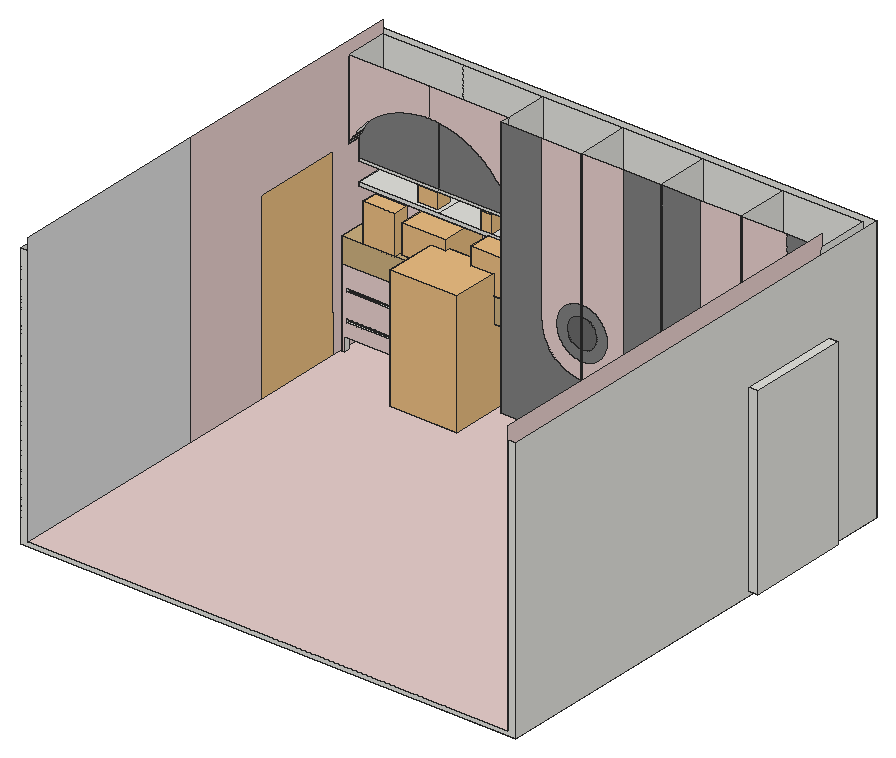
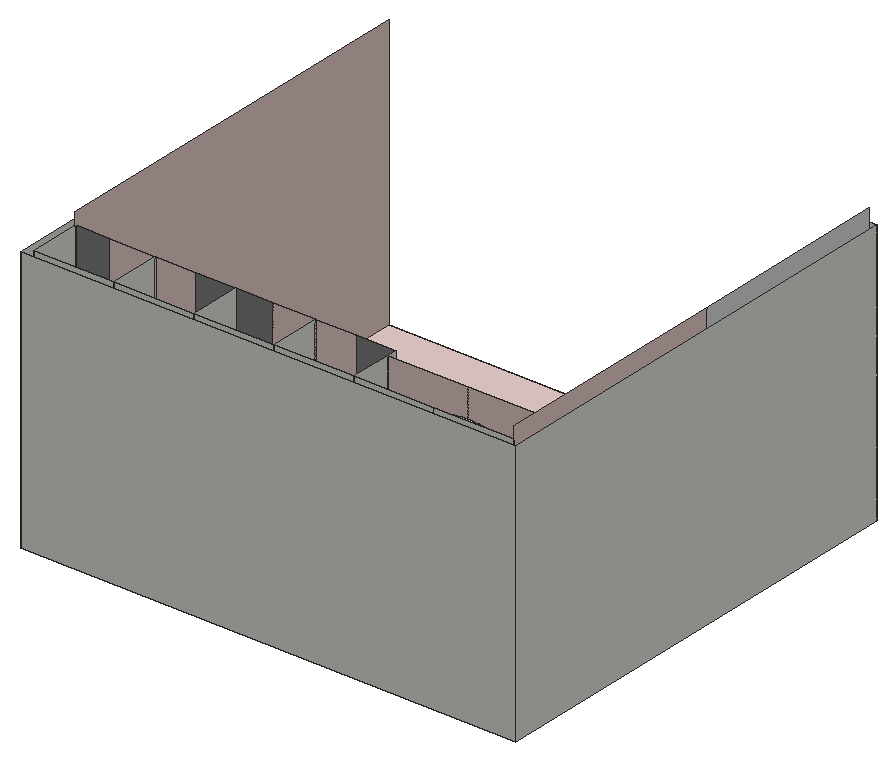
# SketchUp Ruby script. Lengths in inches.
U = 1.inch
M = Sketchup.active_model
def pt(a) = Geom::Point3d.new(a.map { |v| v * U })
def face(e, loops, mat)
  f = e.add_face(loops[0].map { |a| pt(a) })
  loops[1..].each { |l| e.add_face(l.map { |a| pt(a) }).erase! }
  f.material = f.back_material = mat if mat
  f
end
# faces: each face lists its corners as indices into pts; further lists are holes
def faces(e, pts, list, mat = nil) = list.each { |f| face(e, (f[0].is_a?(Array) ? f : [f]).map { |l| l.map { |i| pts[i] } }, mat) }
# xy, xz, yz: faces in a plane at the given z, y or x. An outline is a flat list of corners, or four numbers for a rectangle; further outlines are holes
def ring(l) = l.size == 4 ? [[l[0], l[1]], [l[2], l[1]], [l[2], l[3]], [l[0], l[3]]] : l.each_slice(2).to_a
def flat(e, list, mat, &to3) = list.each { |f| face(e, (f[0].is_a?(Array) ? f : [f]).map { |l| ring(l).map { |u, v| to3.(u, v) } }, mat) }
def xy(e, z, list, mat = nil) = flat(e, list, mat) { |x, y| [x, y, z] }
def xz(e, y, list, mat = nil) = flat(e, list, mat) { |x, z| [x, y, z] }
def yz(e, x, list, mat = nil) = flat(e, list, mat) { |y, z| [x, y, z] }
def lines(e, pts, list) = list.each { |a, b| e.add_line(pt(pts[a]), pt(pts[b])) }
# prism: a flat outline (further loops are holes) pulled along v
def prism(e, loops, v, mat = nil)
  f = face(e, loops, mat); d = Geom::Vector3d.new(v.map { |x| x * U })
  f.pushpull(f.normal.samedirection?(d) ? d.length : -d.length)
end
def box(e, o, s, mat = nil) = prism(e, [[o, [o[0] + s[0], o[1], o[2]], [o[0] + s[0], o[1] + s[1], o[2]], [o[0], o[1] + s[1], o[2]]]], [0, 0, s[2]], mat)
def at(x, y, z, deg = 0) = Geom::Transformation.translation(pt([x, y, z])) * Geom::Transformation.rotation(ORIGIN, Z_AXIS, deg.degrees)
def axes(o, x, y, z) = Geom::Transformation.new([*x, 0, *y, 0, *z, 0, *pt(o).to_a, 1])
def part(name) = M.definitions.add(name)
# library, detail: a bought-in or finely detailed component or shape, given as its bounding box
def library(name, o, s) = part(name).tap { |d| box(d.entities, o, s) }
def detail(e, o, s) = box(e.add_group.entities, o, s)
def put(e, d, t, mat = nil) = e.add_instance(d, t).tap { |i| i.material = mat if mat }
def group(e, t, mat = nil) = e.add_group.tap { |g| g.transformation = t; g.material = mat if mat }.entities
root = M.entities
M.materials.add("[0007_MistyRose]").color = [232, 207, 204]
M.materials.add("[0130_Gainsboro]").color = [220, 220, 220]
M.materials.add("[0133_Gray]").color = [128, 128, 128]
M.materials.add("[0134_DimGray]").color = [105, 105, 105]
M.materials.add("[0136_Charcoal]").color = [35, 35, 35]
M.materials.add("[Wood Floor Light]").color = [204, 176, 127]
c1 = library("skp9D",[0,-0.2,0],[0.48,0.4,0.87])
c2 = part("Group\#2")
detail(c2.entities,[0,0,0],[36,3,84])
c3 = library("Flower+Vase+Glass",[1.07,1.25,0],[13.84,13.38,16.78])
c4 = library("LapTop",[-9.12,-3.35,-0.68],[14.19,15.07,9.17])
c5 = library("Lampe Enna desk ASTRO",[0,0,0],[14.67,7.08,17.81])
c6 = library("ADORNOS+LIVROS+PLANTA+CELULAR+ÓCULOS",[6.19,-1.3125,-0.22],[15.35,11.9,12.07])
c7 = library("Group\#6",[0,0,0],[2.77,2.73,4.26])
xy(root,0,[[0,0,228,207.6875]])
xy(root,2.125,[[3.62,180.25,5.05,183.03],[38.11,180.25,40.45,183.62],[77.27,180.25,114.09,204.25],[114.39,180.25,150.92,180.25,150.92,204.25,114.09,204.25,114.09,180.38,114.39,180.38],[150.92,180.25,187.74,204.25],
  [188.04,180.25,224.57,180.25,224.57,204.25,187.74,204.25,187.74,180.38,188.04,180.38],[3.62,196.71,5.05,196.71,5.05,199.93,40.45,199.93,40.45,204.25,3.62,204.25],[40.45,202.25,77.27,204.25]])
xy(root,2.125,[[[3.43,0,224.57,0,224.57,134,232.38,134,232.38,180.25,188.04,180.25,188.04,180.38,187.74,180.38,187.74,180.25,114.39,180.25,114.39,180.38,114.09,180.38,114.09,180.25,77.27,180.25,77.27,202.25,40.45,202.25,40.45,199.93,5.05,199.93,5.05,196.71,3.62,196.71,3.62,204.25,3.57,175.68,0.14,175.69,0.07,134.44,3.5,134.43,3.43,93.375],[38.11,180.25,40.45,183.62],[3.62,180.25,5.05,183.03]]],"[0007_MistyRose]")
xy(root,8.1875,[[5.05,180.25,5.05,183.03,3.62,183.03,3.62,196.71,5.05,196.71,5.05,199.93,30.74,199.93,30.74,183.62,38.11,183.62,38.11,180.25],[30.74,183.62,40.45,199.93]])
xy(root,14.46,[[5.96,180.25,37.02,181.5]])
xy(root,16.15,[[5.96,180.25,37.02,181.5]])
xy(root,26.96,[[5.96,180.25,37.02,181.5]])
xy(root,28.65,[[5.96,180.25,37.02,181.5]])
xy(root,37.85,[[40.45,180.25,77.27,202.25]])
xy(root,49.45,[[3.62,180.25,77.27,203.88]],"[Wood Floor Light]")
xy(root,65.5,[[3.62,190.13,40.45,203.88],[40.45,190.13,77.27,203.88]])
xy(root,67.29,[[3.62,190.13,40.45,203.88],[40.45,190.13,77.27,203.88]])
xy(root,76.04,[[3.62,190.13,77.27,203.88]])
xy(root,86.125,[[224.57,134,232.38,180.25],[3.5,134.43,0.07,134.44,0.14,175.69,3.57,175.68]])
xz(root,0,[[0,0,228,0,228,122.125,224.57,122.125,224.57,2.125,3.43,2.125,3.43,122.125,0,122.125]])
xz(root,134,[[224.57,2.125,232.38,86.125]])
xz(root,180.25,[[150.92,2.125,151.22,122.125],[114.39,36.55,114.39,41.12,114.09,41.16,114.09,36.59],[187.74,36.6,188.04,36.64,188.04,40.48,187.74,40.44],[187.74,40.44,188.04,40.48,188.04,55.625,187.74,55.67],[114.39,41.12,114.39,54.99,114.09,54.95,114.09,41.16],
  [114.09,54.95,114.39,54.99,114.39,59.55,114.09,59.51],[188.04,55.625,188.04,59.46,187.74,59.5,187.74,55.67]])
xz(root,180.25,[[[3.62,2.125,5.05,2.125,5.05,8.1875,38.11,8.1875,38.11,2.125,40.45,2.125,40.45,37.85,3.62,37.85],[5.96,26.96,37.02,28.65],[5.96,14.46,37.02,16.15]],[224.57,2.125,232.38,86.125],[188.57,28.22,189.1,28.22,189.63,28.23,190.16,28.25,190.6875,28.29,191.21,28.35,191.74,28.41,192.26,28.49,192.79,28.59,193.3,28.7,193.82,28.82,194.33,28.96,194.84,29.11,195.35,29.28,195.85,29.45,196.83,29.85,197.3125,30.07,197.79,30.3,198.26,30.54,198.72,30.8,199.18,31.07,199.63,31.35,200.07,31.64,200.51,31.95,201.35,32.59,201.76,32.93,202.16,33.28,202.55,33.64,203.29,34.4,203.65,34.79,204,35.1875,204.34,35.6,204.98,36.44,205.28,36.88,205.57,37.32,205.85,37.77,206.11,38.23,206.37,38.7,206.61,39.17,206.84,39.65,207.05,40.13,207.26,40.625,207.44,41.12,207.62,41.62,207.78,42.125,207.93,42.63,208.07,43.15,208.1875,43.66,208.29,44.18,208.38,44.71,208.46,45.23,208.53,45.76,208.58,46.29,208.61,46.81,208.63,47.34,208.64,47.875,208.64,122.125,188.04,122.125,188.04,59.46,188.63,59.47,189.22,59.41,189.8,59.32,190.375,59.2,190.95,59.05,191.51,58.87,192.06,58.66,192.6,58.42,193.125,58.16,193.64,57.87,194.14,57.55,194.62,57.21,195.08,56.84,195.52,56.45,195.94,56.04,196.34,55.61,196.72,55.16,197.08,54.6875,197.4,54.2,197.71,53.69,197.98,53.17,198.23,52.64,198.46,52.09,198.65,51.53,198.8125,50.97,198.95,50.39,199.06,49.82,199.13,49.23,199.18,48.64,199.19,48.05,199.18,47.46,199.13,46.875,199.06,46.29,198.95,45.71,198.8125,45.14,198.65,44.57,198.46,44.02,198.23,43.47,197.98,42.9375,197.71,42.42,197.4,41.91,197.08,41.42,196.72,40.95,196.34,40.5,195.94,40.0625,195.52,39.65,195.08,39.26,194.62,38.9,194.14,38.56,193.64,38.24,193.125,37.95,192.6,37.68,192.06,37.45,191.51,37.24,190.95,37.0625,190.375,36.91,189.8,36.79,189.22,36.7,188.63,36.64,188.04,36.64,188.04,28.34],[187.24,28.3,187.74,28.38,187.74,36.6,187.14,36.62,186.54,36.67,185.95,36.74,185.36,36.85,184.78,36.99,184.2,37.16,183.64,37.36,183.08,37.59,182.54,37.85,182.02,38.14,181.51,38.45,181.01,38.79,180.54,39.16,180.08,39.54,179.64,39.96,179.23,40.39,178.84,40.85,178.48,41.32,178.14,41.82,177.83,42.33,177.54,42.86,177.28,43.4,177.05,43.95,176.85,44.52,176.68,45.09,176.54,45.67,176.43,46.26,176.35,46.86,176.31,47.45,176.29,48.05,176.31,48.65,176.35,49.25,176.43,49.84,176.54,50.43,176.68,51.02,176.85,51.59,177.05,52.16,177.28,52.71,177.54,53.25,177.83,53.78,178.14,54.29,178.48,54.78,178.84,55.26,179.23,55.72,179.64,56.15,180.08,56.5625,180.54,56.95,181.01,57.32,181.51,57.66,182.02,57.97,182.54,58.26,183.08,58.51,183.64,58.74,184.2,58.94,184.78,59.11,185.36,59.25,185.95,59.36,186.54,59.44,187.14,59.49,187.74,59.5,187.74,122.125,169.33,122.125,169.33,47.875,169.34,47.38,169.35,46.89,169.39,46.4,169.43,45.9,169.48,45.41,169.55,44.92,169.63,44.4375,169.72,43.95,169.83,43.47,170.07,42.51,170.37,41.57,170.53,41.1,170.71,40.64,170.9,40.1875,171.09,39.73,171.3,39.29,171.76,38.41,172,37.98,172.25,37.56,172.52,37.14,172.79,36.73,173.08,36.33,173.375,35.93,173.68,35.54,173.99,35.16,174.32,34.79,174.65,34.43,174.99,34.07,175.34,33.72,175.7,33.38,176.07,33.06,176.45,32.74,176.83,32.43,177.22,32.125,177.625,31.84,178.03,31.56,178.44,31.29,178.86,31.03,179.29,30.78,179.72,30.54,180.16,30.3125,180.6,30.1,181.05,29.89,181.97,29.51,182.43,29.34,183.37,29.04,183.84,28.9,184.32,28.78,184.8,28.67,185.29,28.57,185.77,28.48,186.26,28.41,186.75,28.35],[114.89,28.5,115.89,28.54,116.39,28.58,116.89,28.64,117.38,28.7,117.875,28.78,118.36,28.875,118.85,28.98,119.34,29.1,119.82,29.23,120.3,29.37,120.77,29.53,121.24,29.7,121.71,29.88,122.17,30.07,123.08,30.49,123.52,30.72,123.96,30.96,124.39,31.21,124.8125,31.48,125.23,31.75,125.64,32.04,126.04,32.33,126.4375,32.64,126.82,32.96,127.2,33.28,127.57,33.62,127.93,33.97,128.28,34.32,128.62,34.6875,128.95,35.0625,129.27,35.44,129.59,35.83,129.89,36.23,130.18,36.64,130.46,37.05,130.72,37.48,130.98,37.9,131.23,38.34,131.46,38.78,131.9,39.68,132.28,40.6,132.62,41.54,132.77,42.02,133.03,42.98,133.14,43.47,133.32,44.45,133.39,44.95,133.45,45.44,133.5,45.94,133.53,46.4375,133.55,46.9375,133.56,47.4375,133.56,122.125,114.39,122.125,114.39,59.55,115,59.54,115.6,59.49,116.19,59.41,116.78,59.3,117.37,59.16,117.95,58.99,118.51,58.79,119.07,58.56,119.61,58.3,120.14,58.01,120.66,57.7,121.15,57.36,121.63,56.99,122.09,56.6,122.53,56.19,122.94,55.75,123.33,55.29,123.7,54.8125,124.04,54.32,124.35,53.8,124.64,53.27,124.9,52.73,125.13,52.17,125.33,51.61,125.5,51.03,125.64,50.44,125.75,49.85,125.83,49.26,125.88,48.66,125.89,48.05,125.88,47.45,125.83,46.85,125.75,46.25,125.64,45.66,125.5,45.08,125.33,44.5,125.13,43.93,124.9,43.375,124.64,42.83,124.35,42.3,124.04,41.79,123.7,41.29,123.33,40.82,122.94,40.36,122.53,39.92,122.09,39.51,121.63,39.12,121.15,38.75,120.66,38.41,120.14,38.09,119.61,37.81,119.07,37.55,118.51,37.32,117.95,37.12,117.37,36.95,116.78,36.8,116.19,36.7,115.6,36.62,115,36.57,114.39,36.55,114.39,28.53],
  [113.61,28.53,114.09,28.57,114.09,36.59,113.5,36.59,112.91,36.65,112.33,36.74,111.75,36.86,111.18,37.01,110.61,37.19,110.06,37.4,109.52,37.64,108.99,37.9,108.47,38.2,107.97,38.51,107.49,38.86,107.02,39.22,106.58,39.62,106.16,40.03,105.75,40.46,105.375,40.92,105.02,41.39,104.6875,41.88,104.38,42.39,104.11,42.91,103.86,43.45,103.63,44,103.4375,44.56,103.27,45.125,103.14,45.7,103.03,46.28,102.95,46.87,102.91,47.46,102.89,48.05,102.91,48.65,102.95,49.24,103.03,49.82,103.14,50.41,103.27,50.98,103.4375,51.55,103.63,52.11,103.86,52.66,104.11,53.19,104.38,53.72,104.6875,54.22,105.02,54.72,105.375,55.1875,105.75,55.64,106.16,56.08,106.58,56.49,107.02,56.88,107.49,57.25,107.97,57.59,108.47,57.91,108.99,58.2,109.52,58.47,110.06,58.7,110.61,58.91,111.18,59.09,111.75,59.25,112.33,59.37,112.91,59.46,113.5,59.52,114.09,59.51,114.09,122.125,95.68,122.125,95.68,47.4375,95.6875,46.95,95.71,46.46,95.74,45.98,95.78,45.49,95.84,45.01,95.91,44.53,95.99,44.05,96.08,43.57,96.1875,43.09,96.3,42.62,96.43,42.15,96.58,41.6875,96.73,41.22,96.9,40.77,97.07,40.3125,97.26,39.86,97.46,39.42,97.67,38.98,98.13,38.12,98.375,37.7,98.63,37.29,98.9,36.88,99.46,36.08,99.76,35.7,100.07,35.32,100.38,34.95,101.04,34.23,101.74,33.55,102.1,33.23,102.47,32.91,102.85,32.6,103.23,32.3,103.625,32.02,104.03,31.74,104.43,31.47,105.27,30.97,105.69,30.73,106.13,30.51,106.57,30.3,107.01,30.1,107.46,29.91,107.91,29.73,108.37,29.5625,108.83,29.41,109.29,29.26,109.76,29.13,110.24,29.01,110.71,28.91,111.1875,28.8125,111.67,28.73,112.15,28.66,112.63,28.6,113.12,28.56]],"[0007_MistyRose]")
xz(root,180.25,[[77.27,2.125,114.09,2.125,114.09,28.57,113.61,28.53,113.12,28.56,112.63,28.6,112.15,28.66,111.67,28.73,111.1875,28.8125,110.71,28.91,110.24,29.01,109.76,29.13,109.29,29.26,108.83,29.41,108.37,29.5625,107.91,29.73,107.46,29.91,107.01,30.1,106.57,30.3,106.13,30.51,105.69,30.73,105.27,30.97,104.43,31.47,104.03,31.74,103.625,32.02,103.23,32.3,102.85,32.6,102.47,32.91,102.1,33.23,101.74,33.55,101.04,34.23,100.38,34.95,100.07,35.32,99.76,35.7,99.46,36.08,98.9,36.88,98.63,37.29,98.375,37.7,98.13,38.12,97.67,38.98,97.46,39.42,97.26,39.86,97.07,40.3125,96.9,40.77,96.73,41.22,96.58,41.6875,96.43,42.15,96.3,42.62,96.1875,43.09,96.08,43.57,95.99,44.05,95.91,44.53,95.84,45.01,95.78,45.49,95.74,45.98,95.71,46.46,95.6875,46.95,95.68,47.4375,95.68,122.125,77.27,122.125],[114.39,2.125,150.92,2.125,150.92,122.125,133.56,122.125,133.56,47.4375,133.55,46.9375,133.53,46.4375,133.5,45.94,133.45,45.44,133.39,44.95,133.32,44.45,133.14,43.47,133.03,42.98,132.77,42.02,132.62,41.54,132.28,40.6,131.9,39.68,131.46,38.78,131.23,38.34,130.98,37.9,130.72,37.48,130.46,37.05,130.18,36.64,129.89,36.23,129.59,35.83,129.27,35.44,128.95,35.0625,128.62,34.6875,128.28,34.32,127.93,33.97,127.57,33.62,127.2,33.28,126.82,32.96,126.4375,32.64,126.04,32.33,125.64,32.04,125.23,31.75,124.8125,31.48,124.39,31.21,123.96,30.96,123.52,30.72,123.08,30.49,122.17,30.07,121.71,29.88,121.24,29.7,120.77,29.53,120.3,29.37,119.82,29.23,119.34,29.1,118.85,28.98,118.36,28.875,117.875,28.78,117.38,28.7,116.89,28.64,116.39,28.58,115.89,28.54,114.89,28.5,114.39,28.53],[151.22,2.125,187.74,2.125,187.74,28.38,187.24,28.3,186.75,28.35,186.26,28.41,185.77,28.48,185.29,28.57,184.8,28.67,184.32,28.78,183.84,28.9,183.37,29.04,182.43,29.34,181.97,29.51,181.05,29.89,180.6,30.1,180.16,30.3125,179.72,30.54,179.29,30.78,178.86,31.03,178.44,31.29,178.03,31.56,177.625,31.84,177.22,32.125,176.83,32.43,176.45,32.74,176.07,33.06,175.7,33.38,175.34,33.72,174.99,34.07,174.65,34.43,174.32,34.79,173.99,35.16,173.68,35.54,173.375,35.93,173.08,36.33,172.79,36.73,172.52,37.14,172.25,37.56,172,37.98,171.76,38.41,171.3,39.29,171.09,39.73,170.9,40.1875,170.71,40.64,170.53,41.1,170.37,41.57,170.07,42.51,169.83,43.47,169.72,43.95,169.63,44.4375,169.55,44.92,169.48,45.41,169.43,45.9,169.39,46.4,169.35,46.89,169.34,47.38,169.33,47.875,169.33,122.125,151.22,122.125],[188.04,2.125,224.57,2.125,224.57,122.125,208.64,122.125,208.64,47.875,208.63,47.34,208.61,46.81,208.58,46.29,208.53,45.76,208.46,45.23,208.38,44.71,208.29,44.18,208.1875,43.66,208.07,43.15,207.93,42.63,207.78,42.125,207.62,41.62,207.44,41.12,207.26,40.625,207.05,40.13,206.84,39.65,206.61,39.17,206.37,38.7,206.11,38.23,205.85,37.77,205.57,37.32,205.28,36.88,204.98,36.44,204.34,35.6,204,35.1875,203.65,34.79,203.29,34.4,202.55,33.64,202.16,33.28,201.76,32.93,201.35,32.59,200.51,31.95,200.07,31.64,199.63,31.35,199.18,31.07,198.72,30.8,198.26,30.54,197.79,30.3,197.3125,30.07,196.83,29.85,195.85,29.45,195.35,29.28,194.84,29.11,194.33,28.96,193.82,28.82,193.3,28.7,192.79,28.59,192.26,28.49,191.74,28.41,191.21,28.35,190.6875,28.29,190.16,28.25,189.63,28.23,189.1,28.22,188.57,28.22,188.04,28.34],[114.39,36.55,115,36.57,115.6,36.62,116.19,36.7,116.78,36.8,117.37,36.95,117.95,37.12,118.51,37.32,119.07,37.55,119.61,37.81,120.14,38.09,120.66,38.41,121.15,38.75,121.63,39.12,122.09,39.51,122.53,39.92,122.94,40.36,123.33,40.82,123.7,41.29,124.04,41.79,124.35,42.3,124.64,42.83,124.9,43.375,125.13,43.93,125.33,44.5,125.5,45.08,125.64,45.66,125.75,46.25,125.83,46.85,125.88,47.45,125.89,48.05,125.88,48.66,125.83,49.26,125.75,49.85,125.64,50.44,125.5,51.03,125.33,51.61,125.13,52.17,124.9,52.73,124.64,53.27,124.35,53.8,124.04,54.32,123.7,54.8125,123.33,55.29,122.94,55.75,122.53,56.19,122.09,56.6,121.63,56.99,121.15,57.36,120.66,57.7,120.14,58.01,119.61,58.3,119.07,58.56,118.51,58.79,117.95,58.99,117.37,59.16,116.78,59.3,116.19,59.41,115.6,59.49,115,59.54,114.39,59.55,114.39,54.99,114.76,54.98,115.12,54.95,115.48,54.91,115.84,54.84,116.1875,54.75,116.54,54.65,116.88,54.53,117.22,54.39,117.54,54.23,117.86,54.0625,118.17,53.87,118.47,53.67,118.76,53.45,119.04,53.21,119.3,52.96,119.55,52.7,119.79,52.42,120.01,52.13,120.21,51.83,120.4,51.52,120.58,51.2,120.73,50.875,120.87,50.54,120.99,50.2,121.09,49.85,121.18,49.5,121.25,49.14,121.29,48.78,121.32,48.42,121.33,48.05,121.32,47.69,121.29,47.33,121.25,46.97,121.18,46.61,121.09,46.26,120.99,45.91,120.87,45.57,120.73,45.23,120.58,44.9,120.4,44.58,120.21,44.28,120.01,43.98,119.79,43.6875,119.55,43.41,119.3,43.15,119.04,42.9,118.76,42.66,118.47,42.44,118.17,42.24,117.86,42.05,117.54,41.87,117.22,41.72,116.88,41.58,116.54,41.46,116.1875,41.35,115.84,41.27,115.48,41.2,115.12,41.15,114.76,41.125,114.39,41.12],
  [113.5,36.59,114.09,36.59,114.09,41.16,113.74,41.15,113.39,41.1875,113.04,41.25,112.7,41.33,112.36,41.42,112.02,41.53,111.69,41.66,111.37,41.81,111.06,41.97,110.75,42.15,110.46,42.34,110.17,42.55,109.9,42.77,109.63,43.01,109.38,43.26,109.15,43.52,108.92,43.79,108.71,44.07,108.52,44.37,108.34,44.67,108.17,44.98,108.02,45.31,107.89,45.63,107.78,45.97,107.68,46.31,107.6,46.65,107.54,47,107.49,47.35,107.47,47.7,107.46,48.05,107.47,48.41,107.49,48.76,107.54,49.11,107.6,49.46,107.68,49.8,107.78,50.14,107.89,50.47,108.02,50.8,108.17,51.12,108.34,51.43,108.52,51.74,108.71,52.03,108.92,52.32,109.15,52.59,109.38,52.85,109.63,53.1,109.9,53.34,110.17,53.56,110.46,53.77,110.75,53.96,111.06,54.14,111.37,54.3,111.69,54.44,112.02,54.57,112.36,54.69,112.7,54.78,113.04,54.86,113.39,54.92,113.74,54.96,114.09,54.95,114.09,59.51,113.5,59.52,112.91,59.46,112.33,59.37,111.75,59.25,111.18,59.09,110.61,58.91,110.06,58.7,109.52,58.47,108.99,58.2,108.47,57.91,107.97,57.59,107.49,57.25,107.02,56.88,106.58,56.49,106.16,56.08,105.75,55.64,105.375,55.1875,105.02,54.72,104.6875,54.22,104.38,53.72,104.11,53.19,103.86,52.66,103.63,52.11,103.4375,51.55,103.27,50.98,103.14,50.41,103.03,49.82,102.95,49.24,102.91,48.65,102.89,48.05,102.91,47.46,102.95,46.87,103.03,46.28,103.14,45.7,103.27,45.125,103.4375,44.56,103.63,44,103.86,43.45,104.11,42.91,104.38,42.39,104.6875,41.88,105.02,41.39,105.375,40.92,105.75,40.46,106.16,40.03,106.58,39.62,107.02,39.22,107.49,38.86,107.97,38.51,108.47,38.2,108.99,37.9,109.52,37.64,110.06,37.4,110.61,37.19,111.18,37.01,111.75,36.86,112.33,36.74,112.91,36.65],[187.74,36.6,187.74,40.44,187.34,40.45,186.95,40.48,186.55,40.54,186.16,40.61,185.77,40.7,185.39,40.81,185.01,40.95,184.65,41.1,184.29,41.27,183.9375,41.46,183.6,41.67,183.27,41.9,182.95,42.14,182.65,42.4,182.36,42.67,182.08,42.96,181.83,43.26,181.58,43.58,181.36,43.91,181.15,44.25,180.96,44.6,180.79,44.96,180.64,45.33,180.5,45.7,180.39,46.08,180.3,46.47,180.22,46.86,180.17,47.26,180.14,47.66,180.13,48.05,180.14,48.45,180.17,48.85,180.22,49.24,180.3,49.64,180.39,50.02,180.5,50.41,180.64,50.78,180.79,51.15,180.96,51.51,181.15,51.86,181.36,52.2,181.58,52.53,182.08,53.15,182.36,53.4375,182.65,53.71,182.95,53.97,183.27,54.21,183.6,54.4375,183.9375,54.65,184.29,54.84,184.65,55.01,185.01,55.16,185.39,55.29,185.77,55.41,186.16,55.5,186.55,55.57,186.95,55.625,187.34,55.65,187.74,55.67,187.74,59.5,187.14,59.49,186.54,59.44,185.95,59.36,185.36,59.25,184.78,59.11,184.2,58.94,183.64,58.74,183.08,58.51,182.54,58.26,182.02,57.97,181.51,57.66,181.01,57.32,180.54,56.95,180.08,56.5625,179.64,56.15,179.23,55.72,178.84,55.26,178.48,54.78,178.14,54.29,177.83,53.78,177.54,53.25,177.28,52.71,177.05,52.16,176.85,51.59,176.68,51.02,176.54,50.43,176.43,49.84,176.35,49.25,176.31,48.65,176.29,48.05,176.31,47.45,176.35,46.86,176.43,46.26,176.54,45.67,176.68,45.09,176.85,44.52,177.05,43.95,177.28,43.4,177.54,42.86,177.83,42.33,178.14,41.82,178.48,41.32,178.84,40.85,179.23,40.39,179.64,39.96,180.08,39.54,180.54,39.16,181.01,38.79,181.51,38.45,182.02,38.14,182.54,37.85,183.08,37.59,183.64,37.36,184.2,37.16,184.78,36.99,185.36,36.85,185.95,36.74,186.54,36.67,187.14,36.62],[188.04,36.64,188.63,36.64,189.22,36.7,189.8,36.79,190.375,36.91,190.95,37.0625,191.51,37.24,192.06,37.45,192.6,37.68,193.125,37.95,193.64,38.24,194.14,38.56,194.62,38.9,195.08,39.26,195.52,39.65,195.94,40.0625,196.34,40.5,196.72,40.95,197.08,41.42,197.4,41.91,197.71,42.42,197.98,42.9375,198.23,43.47,198.46,44.02,198.65,44.57,198.8125,45.14,198.95,45.71,199.06,46.29,199.13,46.875,199.18,47.46,199.19,48.05,199.18,48.64,199.13,49.23,199.06,49.82,198.95,50.39,198.8125,50.97,198.65,51.53,198.46,52.09,198.23,52.64,197.98,53.17,197.71,53.69,197.4,54.2,197.08,54.6875,196.72,55.16,196.34,55.61,195.94,56.04,195.52,56.45,195.08,56.84,194.62,57.21,194.14,57.55,193.64,57.87,193.125,58.16,192.6,58.42,192.06,58.66,191.51,58.87,190.95,59.05,190.375,59.2,189.8,59.32,189.22,59.41,188.63,59.47,188.04,59.46,188.04,55.625,188.43,55.63,188.82,55.59,189.2,55.52,189.58,55.44,189.95,55.34,190.32,55.21,190.68,55.07,191.04,54.91,191.38,54.74,191.72,54.54,192.05,54.33,192.36,54.1,192.66,53.86,192.95,53.6,193.23,53.33,193.49,53.04,193.74,52.74,193.97,52.43,194.18,52.11,194.38,51.77,194.5625,51.43,194.73,51.08,194.87,50.72,195,50.35,195.11,49.98,195.19,49.6,195.26,49.21,195.3125,48.83,195.34,48.44,195.35,48.05,195.34,47.67,195.3125,47.28,195.26,46.89,195.19,46.51,195.11,46.13,195,45.76,194.87,45.39,194.73,45.03,194.5625,44.68,194.38,44.34,194.18,44,193.97,43.68,193.74,43.37,193.49,43.07,193.23,42.78,192.95,42.51,192.66,42.25,192.36,42,192.05,41.78,191.72,41.5625,191.38,41.37,191.04,41.19,190.68,41.03,190.32,40.89,189.95,40.77,189.58,40.67,189.2,40.58,188.82,40.52,188.43,40.47,188.04,40.48]],"[0133_Gray]")
xz(root,180.25,[[187.74,40.44,187.74,55.67,187.34,55.65,186.95,55.625,186.55,55.57,186.16,55.5,185.77,55.41,185.39,55.29,185.01,55.16,184.65,55.01,184.29,54.84,183.9375,54.65,183.6,54.4375,183.27,54.21,182.95,53.97,182.65,53.71,182.36,53.4375,182.08,53.15,181.58,52.53,181.36,52.2,181.15,51.86,180.96,51.51,180.79,51.15,180.64,50.78,180.5,50.41,180.39,50.02,180.3,49.64,180.22,49.24,180.17,48.85,180.14,48.45,180.13,48.05,180.14,47.66,180.17,47.26,180.22,46.86,180.3,46.47,180.39,46.08,180.5,45.7,180.64,45.33,180.79,44.96,180.96,44.6,181.15,44.25,181.36,43.91,181.58,43.58,181.83,43.26,182.08,42.96,182.36,42.67,182.65,42.4,182.95,42.14,183.27,41.9,183.6,41.67,183.9375,41.46,184.29,41.27,184.65,41.1,185.01,40.95,185.39,40.81,185.77,40.7,186.16,40.61,186.55,40.54,186.95,40.48,187.34,40.45],[188.43,40.47,188.82,40.52,189.2,40.58,189.58,40.67,189.95,40.77,190.32,40.89,190.68,41.03,191.04,41.19,191.38,41.37,191.72,41.5625,192.05,41.78,192.36,42,192.66,42.25,192.95,42.51,193.23,42.78,193.49,43.07,193.74,43.37,193.97,43.68,194.18,44,194.38,44.34,194.5625,44.68,194.73,45.03,194.87,45.39,195,45.76,195.11,46.13,195.19,46.51,195.26,46.89,195.3125,47.28,195.34,47.67,195.35,48.05,195.34,48.44,195.3125,48.83,195.26,49.21,195.19,49.6,195.11,49.98,195,50.35,194.87,50.72,194.73,51.08,194.5625,51.43,194.38,51.77,194.18,52.11,193.97,52.43,193.74,52.74,193.49,53.04,193.23,53.33,192.95,53.6,192.66,53.86,192.36,54.1,192.05,54.33,191.72,54.54,191.38,54.74,191.04,54.91,190.68,55.07,190.32,55.21,189.95,55.34,189.58,55.44,189.2,55.52,188.82,55.59,188.43,55.63,188.04,55.625,188.04,40.48],[114.39,41.12,114.76,41.125,115.12,41.15,115.48,41.2,115.84,41.27,116.1875,41.35,116.54,41.46,116.88,41.58,117.22,41.72,117.54,41.87,117.86,42.05,118.17,42.24,118.47,42.44,118.76,42.66,119.04,42.9,119.3,43.15,119.55,43.41,119.79,43.6875,120.01,43.98,120.21,44.28,120.4,44.58,120.58,44.9,120.73,45.23,120.87,45.57,120.99,45.91,121.09,46.26,121.18,46.61,121.25,46.97,121.29,47.33,121.32,47.69,121.33,48.05,121.32,48.42,121.29,48.78,121.25,49.14,121.18,49.5,121.09,49.85,120.99,50.2,120.87,50.54,120.73,50.875,120.58,51.2,120.4,51.52,120.21,51.83,120.01,52.13,119.79,52.42,119.55,52.7,119.3,52.96,119.04,53.21,118.76,53.45,118.47,53.67,118.17,53.87,117.86,54.0625,117.54,54.23,117.22,54.39,116.88,54.53,116.54,54.65,116.1875,54.75,115.84,54.84,115.48,54.91,115.12,54.95,114.76,54.98,114.39,54.99],[113.74,41.15,114.09,41.16,114.09,54.95,113.74,54.96,113.39,54.92,113.04,54.86,112.7,54.78,112.36,54.69,112.02,54.57,111.69,54.44,111.37,54.3,111.06,54.14,110.75,53.96,110.46,53.77,110.17,53.56,109.9,53.34,109.63,53.1,109.38,52.85,109.15,52.59,108.92,52.32,108.71,52.03,108.52,51.74,108.34,51.43,108.17,51.12,108.02,50.8,107.89,50.47,107.78,50.14,107.68,49.8,107.6,49.46,107.54,49.11,107.49,48.76,107.47,48.41,107.46,48.05,107.47,47.7,107.49,47.35,107.54,47,107.6,46.65,107.68,46.31,107.78,45.97,107.89,45.63,108.02,45.31,108.17,44.98,108.34,44.67,108.52,44.37,108.71,44.07,108.92,43.79,109.15,43.52,109.38,43.26,109.63,43.01,109.9,42.77,110.17,42.55,110.46,42.34,110.75,42.15,111.06,41.97,111.37,41.81,111.69,41.66,112.02,41.53,112.36,41.42,112.7,41.33,113.04,41.25,113.39,41.1875]],"[0134_DimGray]")
xz(root,180.25,[[3.62,37.85,40.45,49.45],[40.45,37.85,77.27,49.45]],"[Wood Floor Light]")
xz(root,180.38,[[114.09,2.125,114.39,2.125,114.39,28.53,114.09,28.57],[187.74,2.125,188.04,2.125,188.04,28.34,187.74,28.38],[188.04,28.34,188.04,122.125,187.74,122.125,187.74,28.38],[114.39,28.53,114.39,122.125,114.09,122.125,114.09,28.57]])
xz(root,181.5,[[5.96,14.46,37.02,16.15],[5.96,26.96,37.02,28.65]],"[0136_Charcoal]")
xz(root,183.03,[[3.62,2.125,5.05,8.1875]])
xz(root,183.62,[[38.11,2.125,40.45,8.1875]])
xz(root,184.57,[[3.62,85.39,3.95,86.09,4.29,86.78,4.65,87.46,5.02,88.14,5.4,88.8,5.79,89.47,6.2,90.12,6.62,90.77,7.05,91.4,7.49,92.03,7.94,92.65,8.41,93.27,8.89,93.87,9.375,94.46,9.875,95.05,10.39,95.625,10.91,96.1875,11.44,96.74,11.98,97.29,13.1,98.35,13.67,98.86,14.85,99.86,15.45,100.34,16.06,100.8,16.68,101.26,17.31,101.71,17.94,102.14,18.59,102.56,19.24,102.97,19.9,103.36,20.57,103.75,21.24,104.12,21.92,104.48,22.61,104.82,23.3,105.15,24,105.47,24.71,105.78,25.42,106.07,26.14,106.35,26.86,106.61,27.59,106.86,28.32,107.1,29.06,107.32,29.8,107.53,30.54,107.73,31.29,107.91,32.04,108.07,32.8,108.23,33.55,108.37,34.3125,108.49,35.08,108.6,35.84,108.69,36.6,108.77,37.37,108.84,38.14,108.89,38.91,108.93,39.68,108.95,40.45,108.95,40.45,122.125,3.62,122.125],[77.27,85.39,77.27,122.125,40.45,122.125,40.45,108.95,41.22,108.95,41.98,108.93,42.75,108.89,43.52,108.84,44.29,108.77,45.05,108.69,45.82,108.6,46.58,108.49,47.34,108.37,48.1,108.23,49.6,107.91,50.35,107.73,51.09,107.53,51.83,107.32,52.57,107.1,53.3,106.86,54.03,106.61,54.75,106.35,55.47,106.07,56.18,105.78,56.89,105.47,57.59,105.15,58.28,104.82,58.97,104.48,59.65,104.12,60.33,103.75,61.65,102.97,62.3,102.56,62.95,102.14,63.58,101.71,64.21,101.26,64.83,100.8,65.44,100.34,66.04,99.86,66.64,99.36,67.22,98.86,67.79,98.35,68.36,97.82,68.91,97.29,69.45,96.74,69.98,96.1875,70.51,95.625,71.02,95.05,71.52,94.46,72.01,93.87,72.48,93.27,72.95,92.65,73.4,92.03,73.85,91.4,74.28,90.77,74.7,90.12,75.1,89.47,75.49,88.8,75.875,88.14,76.24,87.46,76.6,86.78,76.94,86.09]],"[0007_MistyRose]")
xz(root,190.13,[[3.62,65.5,77.27,67.29],[3.62,76.04,77.27,77.2],[40.45,77.2,40.75,108.95]])
xz(root,190.13,[[3.62,77.2,40.45,77.2,40.45,108.95,39.68,108.95,38.91,108.93,38.14,108.89,37.37,108.84,36.6,108.77,35.84,108.69,35.08,108.6,34.3125,108.49,33.55,108.37,32.8,108.23,32.04,108.07,31.29,107.91,30.54,107.73,29.8,107.53,29.06,107.32,28.32,107.1,27.59,106.86,26.86,106.61,26.14,106.35,25.42,106.07,24.71,105.78,24,105.47,23.3,105.15,22.61,104.82,21.92,104.48,21.24,104.12,20.57,103.75,19.9,103.36,19.24,102.97,18.59,102.56,17.94,102.14,17.31,101.71,16.68,101.26,16.06,100.8,15.45,100.34,14.85,99.86,13.67,98.86,13.1,98.35,11.98,97.29,11.44,96.74,10.91,96.1875,10.39,95.625,9.875,95.05,9.375,94.46,8.89,93.87,8.41,93.27,7.94,92.65,7.49,92.03,7.05,91.4,6.62,90.77,6.2,90.12,5.79,89.47,5.4,88.8,5.02,88.14,4.65,87.46,4.29,86.78,3.95,86.09,3.62,85.39],[40.75,77.2,77.27,77.2,77.27,85.39,76.94,86.09,76.6,86.78,76.24,87.46,75.875,88.14,75.49,88.8,75.1,89.47,74.7,90.12,74.28,90.77,73.85,91.4,73.4,92.03,72.95,92.65,72.48,93.27,72.01,93.87,71.52,94.46,71.02,95.05,70.51,95.625,69.98,96.1875,69.45,96.74,68.91,97.29,68.36,97.82,67.79,98.35,67.22,98.86,66.64,99.36,66.04,99.86,65.44,100.34,64.83,100.8,64.21,101.26,63.58,101.71,62.95,102.14,62.3,102.56,61.65,102.97,60.33,103.75,59.65,104.12,58.97,104.48,58.28,104.82,57.59,105.15,56.89,105.47,56.18,105.78,55.47,106.07,54.75,106.35,54.03,106.61,53.3,106.86,52.57,107.1,51.83,107.32,51.09,107.53,50.35,107.73,49.6,107.91,48.1,108.23,47.34,108.37,46.58,108.49,45.82,108.6,45.05,108.69,44.29,108.77,43.52,108.84,42.75,108.89,41.98,108.93,41.22,108.95,40.75,108.95]],"[0133_Gray]")
xz(root,196.71,[[3.62,2.125,5.05,8.1875]])
xz(root,199.93,[[5.05,2.125,38.11,8.1875],[38.11,2.125,40.45,8.1875]])
xz(root,202.25,[[40.45,2.125,77.27,37.85]])
xz(root,203.88,[[3.62,49.45,77.27,65.5],[3.62,67.29,77.27,76.04]],"[0007_MistyRose]")
xz(root,204.25,[[3.62,2.125,40.45,122.125],[40.45,2.125,77.27,122.125],[77.27,2.125,114.09,122.125],[114.09,2.125,150.92,122.125],[150.92,2.125,187.74,122.125],
  [187.74,2.125,224.57,122.125]])
xz(root,207.6875,[[0,0,228,122.125]])
yz(root,0,[[0,0,207.6875,122.125]])
yz(root,3.43,[[0,2.125,93.375,127.75]],"[0130_Gainsboro]")
yz(root,3.62,[[180.25,2.125,180.25,49.45,203.88,49.45,203.88,65.5,190.13,65.5,190.13,67.29,203.88,67.29,203.88,76.04,190.13,76.04,190.13,85.39,184.57,85.39,184.57,122.125,204.25,122.125,204.25,2.125,196.71,2.125,196.71,8.1875,183.03,8.1875,183.03,2.125]])
yz(root,5.05,[[180.25,2.125,183.03,8.1875],[196.71,2.125,199.93,8.1875]])
yz(root,5.96,[[180.25,14.46,181.5,16.15],[180.25,26.96,181.5,28.65]])
yz(root,37.02,[[180.25,14.46,181.5,16.15],[180.25,26.96,181.5,28.65]])
yz(root,38.11,[[180.25,2.125,183.62,8.1875]])
yz(root,40.45,[[180.25,2.125,183.62,2.125,183.62,8.1875,199.93,8.1875,199.93,2.125,202.25,2.125,202.25,37.85,180.25,37.85]])
yz(root,77.27,[[180.25,2.125,202.25,37.85],[202.25,2.125,202.25,37.85,180.25,37.85,180.25,49.45,203.88,49.45,203.88,65.5,190.13,65.5,190.13,67.29,203.88,67.29,203.88,76.04,190.13,76.04,190.13,85.39,184.57,85.39,184.57,122.125,204.25,122.125,204.25,2.125],[180.25,49.45,180.25,122.125,184.57,122.125,184.57,85.39,190.13,85.39,190.13,76.04,203.88,76.04,203.88,67.29,190.13,67.29,190.13,65.5,203.88,65.5,203.88,49.45]])
yz(root,114.09,[[180.25,2.125,180.38,28.57],[180.38,2.125,204.25,122.125],[180.25,28.57,180.38,122.125]])
yz(root,114.39,[[180.25,2.125,180.38,28.53],[180.25,28.53,180.38,28.57],[180.25,28.57,180.38,122.125]])
yz(root,150.92,[[180.25,2.125,204.25,122.125]])
yz(root,187.74,[[180.25,2.125,180.38,28.38],[180.38,2.125,204.25,122.125],[180.25,28.38,180.38,122.125]])
yz(root,188.04,[[180.25,2.125,180.38,28.34],[180.25,28.34,180.38,28.38],[180.25,28.38,180.38,122.125]])
yz(root,224.57,[[180.25,2.125,204.25,122.125]])
yz(root,224.57,[[0,2.125,0,127.75,180.38,127.75,180.38,122.125,180.25,122.125,180.25,86.125,134,86.125,134,2.125]],"[0007_MistyRose]")
yz(root,228,[[0,0,207.6875,122.125]])
yz(root,232.38,[[134,2.125,180.25,86.125]])
p = [[3.62,204.25,2.125],[3.62,204.25,122.125],[3.62,204.25,127.75],[3.43,93.375,127.75],[3.43,93.375,2.125],[3.5,134.43,2.125],
  [3.5,134.43,86.125],[3.57,175.68,86.125],[3.57,175.68,2.125],[0.07,134.44,2.125],[0.14,175.69,2.125],[0.14,175.69,86.125],
  [0.07,134.44,86.125],[3.62,184.57,85.39],[3.62,190.13,85.39],[3.95,190.13,86.09],[3.95,184.57,86.09],[76.94,184.57,86.09],
  [76.94,190.13,86.09],[77.27,190.13,85.39],[77.27,184.57,85.39],[4.29,190.13,86.78],[4.29,184.57,86.78],[76.6,184.57,86.78],
  [76.6,190.13,86.78],[4.65,190.13,87.46],[4.65,184.57,87.46],[76.24,184.57,87.46],[76.24,190.13,87.46],[5.02,190.13,88.14],
  [5.02,184.57,88.14],[75.875,184.57,88.14],[75.875,190.13,88.14],[5.4,190.13,88.8],[5.4,184.57,88.8],[75.49,184.57,88.8],
  [75.49,190.13,88.8],[5.79,190.13,89.47],[5.79,184.57,89.47],[75.1,184.57,89.47],[75.1,190.13,89.47],[6.2,190.13,90.12],
  [6.2,184.57,90.12],[74.7,184.57,90.12],[74.7,190.13,90.12]]
faces(root,p,[[0,1,2,3,4,5,6,7,8]],"[0007_MistyRose]")
faces(root,p,[[9,10,11,12],[12,6,5,9],[10,8,7,11],[13,14,15,16],[17,18,19,20],[16,15,21,22],[23,24,18,17],[22,21,25,26],
  [27,28,24,23],[26,25,29,30],[31,32,28,27],[30,29,33,34],[35,36,32,31],[34,33,37,38],[39,40,36,35],[38,37,41,42],
  [43,44,40,39]])
put(root,c1,axes([42.67,172.12,2.125],[64.52953,0,0],[0,-64.52953,0],[0,0,64.52953]),"[0007_MistyRose]")
put(root,c2,axes([3.57,134.43,2.125],[0,1.14583,0],[-1,0,0],[0,0,1]),"[0007_MistyRose]")
put(root,c2,axes([224.57,175.25,2.125],[0,-1.14583,0],[1,0,0],[0,0,1]),"[0007_MistyRose]")
put(root,c3,at(62.36,179,49.45))
put(root,c4,axes([42.23,187.79,50.42],[1.4238,0,0],[0,1.4238,0],[0,0,1.4238]))
put(root,c5,at(13.65,180.25,49.45))
put(root,c6,axes([25.8,192.95,67.2],[0.58,0,0],[0,0.58,0],[0,0,0.58]))
put(root,c7,axes([59.9,190.13,67.29],[1.84,0,0],[0,1.84,0],[0,0,1.84]))
